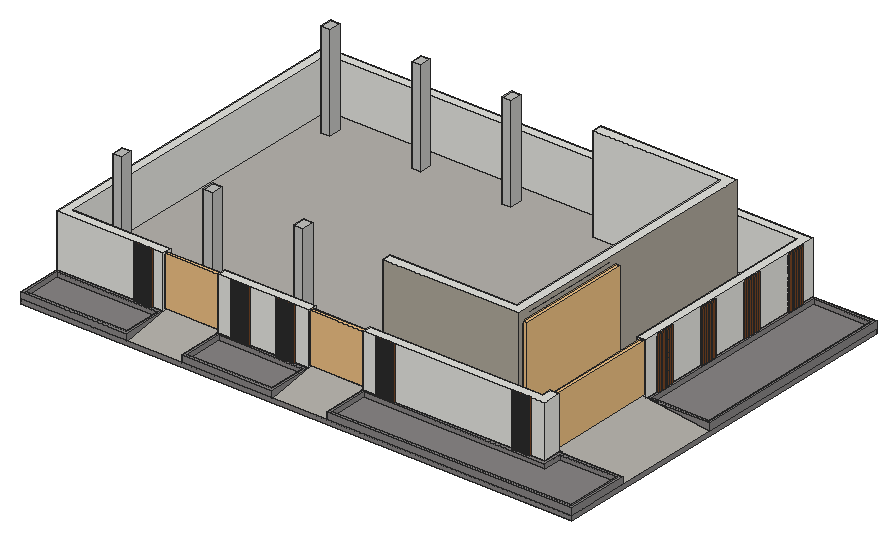
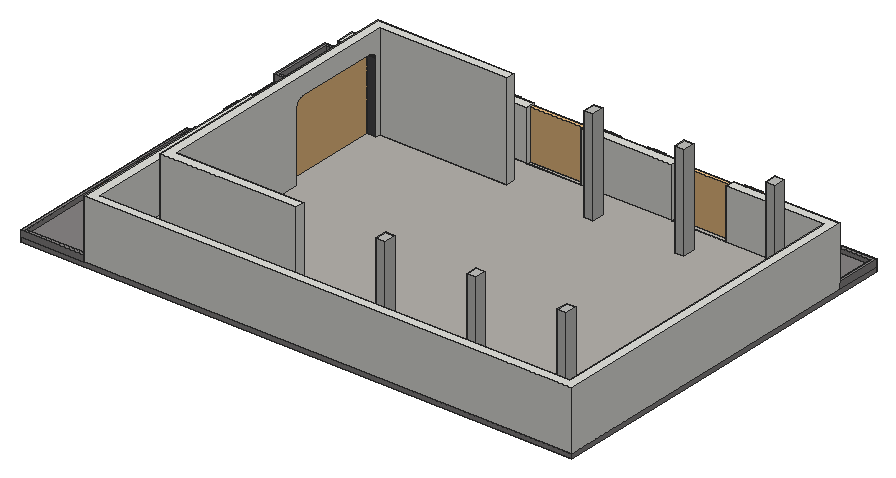
# SketchUp Ruby script. Lengths in inches.
U = 1.inch
M = Sketchup.active_model
def pt(a) = Geom::Point3d.new(a.map { |v| v * U })
def face(e, loops, mat)
  f = e.add_face(loops[0].map { |a| pt(a) })
  loops[1..].each { |l| e.add_face(l.map { |a| pt(a) }).erase! }
  f.material = f.back_material = mat if mat
  f
end
# faces: each face lists its corners as indices into pts; further lists are holes
def faces(e, pts, list, mat = nil) = list.each { |f| face(e, (f[0].is_a?(Array) ? f : [f]).map { |l| l.map { |i| pts[i] } }, mat) }
# xy, xz, yz: faces in a plane at the given z, y or x. An outline is a flat list of corners, or four numbers for a rectangle; further outlines are holes
def ring(l) = l.size == 4 ? [[l[0], l[1]], [l[2], l[1]], [l[2], l[3]], [l[0], l[3]]] : l.each_slice(2).to_a
def flat(e, list, mat, &to3) = list.each { |f| face(e, (f[0].is_a?(Array) ? f : [f]).map { |l| ring(l).map { |u, v| to3.(u, v) } }, mat) }
def xy(e, z, list, mat = nil) = flat(e, list, mat) { |x, y| [x, y, z] }
def xz(e, y, list, mat = nil) = flat(e, list, mat) { |x, z| [x, y, z] }
def yz(e, x, list, mat = nil) = flat(e, list, mat) { |y, z| [x, y, z] }
def lines(e, pts, list) = list.each { |a, b| e.add_line(pt(pts[a]), pt(pts[b])) }
# prism: a flat outline (further loops are holes) pulled along v
def prism(e, loops, v, mat = nil)
  f = face(e, loops, mat); d = Geom::Vector3d.new(v.map { |x| x * U })
  f.pushpull(f.normal.samedirection?(d) ? d.length : -d.length)
end
def box(e, o, s, mat = nil) = prism(e, [[o, [o[0] + s[0], o[1], o[2]], [o[0] + s[0], o[1] + s[1], o[2]], [o[0], o[1] + s[1], o[2]]]], [0, 0, s[2]], mat)
def at(x, y, z, deg = 0) = Geom::Transformation.translation(pt([x, y, z])) * Geom::Transformation.rotation(ORIGIN, Z_AXIS, deg.degrees)
def axes(o, x, y, z) = Geom::Transformation.new([*x, 0, *y, 0, *z, 0, *pt(o).to_a, 1])
def part(name) = M.definitions.add(name)
# library, detail: a bought-in or finely detailed component or shape, given as its bounding box
def library(name, o, s) = part(name).tap { |d| box(d.entities, o, s) }
def detail(e, o, s) = box(e.add_group.entities, o, s)
def put(e, d, t, mat = nil) = e.add_instance(d, t).tap { |i| i.material = mat if mat }
def group(e, t, mat = nil) = e.add_group.tap { |g| g.transformation = t; g.material = mat if mat }.entities
root = M.entities
M.materials.add("1432 AP 8245 TAR ROAD").color = [71, 72, 75]
M.materials.add("Generic").color = [172, 166, 153]
M.materials.add("W142X827B75_NILAYA IMAGINE 31756 ROLL B75").color = [192, 192, 189]
M.materials.add("[Brick Tumbled]").color = [135, 132, 132]
M.materials.add("[Tile Travertine 2 inch]").color = [181, 178, 172]
M.materials.add("[Wood Veneer 01]").color = [120, 70, 37]
c1 = part("Group128\#1")
box(c1.entities,[-12,-39,0],[2,78,1.5])
c2 = part("Group129\#1")
box(c2.entities,[-9.25,-39,0],[2,78,1.5])
c3 = part("Group130\#1")
box(c3.entities,[-6.5,-39,0],[2,78,1.5])
c4 = part("Group131\#1")
box(c4.entities,[-3.75,-39,0],[2,78,1.5])
c5 = part("Group132\#1")
box(c5.entities,[-1,-39,0],[2,78,1.5])
c6 = part("Group133\#1")
box(c6.entities,[1.75,-39,0],[2,78,1.5])
c7 = part("Group134\#1")
box(c7.entities,[4.5,-39,0],[2,78,1.5])
c8 = part("Group135\#1")
box(c8.entities,[7.25,-39,0],[2,78,1.5])
c9 = part("Group136\#1")
box(c9.entities,[10,-39,0],[2,78,1.5])
c10 = part("Group126\#1")
put(c10.entities,c1,at(0,0,0))
put(c10.entities,c2,at(0,0,0))
put(c10.entities,c3,at(0,0,0))
put(c10.entities,c4,at(0,0,0))
put(c10.entities,c5,at(0,0,0))
put(c10.entities,c6,at(0,0,0))
put(c10.entities,c7,at(0,0,0))
put(c10.entities,c8,at(0,0,0))
put(c10.entities,c9,at(0,0,0))
c11 = part("Group\#64")
put(c11.entities,c10,axes([12,0,39],[1,0,0],[0,0,1],[0,-1,0]))
c12 = part("Group\#66")
prism(c12.entities,[[[0,-72,0],[0,0,12],[0,0,0]]],[72,0,0])
c13 = library("Group\#1077",[59.37,-1.74,0],[60.38,4.74,59.75])
c14 = library("Group\#63",[0,7,0],[5,154,113])
c15 = library("Double slatted gate",[7.03,-128.55,-3.91],[5.33,99.02,60.06])
c16 = part("5")
box(c16.entities,[0,0,0],[12,16,126])
box(root,[0,0,11.79],[729,503.37,6],"[Brick Tumbled]")
g1 = group(root,at(0,0,17.79),"[Brick Tumbled]")
xy(g1,0,[[0,0,141,60],[213,0,333,60],[405,0,405,60,645,60,645,84,729,84,729,0],[645,228,729,503.37]])
xy(g1,3,[[4,4,137,56],[217,4,329,56],[409,4,725,4,725,80,649,80,649,56,409,56],[649,232,725,499.37]])
xy(g1,9,[[[0,0,141,60],[4,4,137,56]],[[213,0,333,60],[217,4,329,56]],[[405,0,729,0,729,84,645,84,645,60,405,60],[409,4,409,56,649,56,649,80,725,80,725,4]],[[645,228,729,503.37],[649,232,725,499.37]]])
xz(g1,0,[[0,0,141,9],[213,0,333,9],[405,0,729,9]])
xz(g1,4,[[4,3,137,9],[217,3,329,9],[409,3,725,9]])
xz(g1,56,[[4,3,137,9],[217,3,329,9],[409,3,649,9]])
xz(g1,60,[[0,0,141,9],[213,0,333,9],[405,0,645,9]])
xz(g1,80,[[649,3,725,9]])
xz(g1,84,[[645,0,729,9]])
xz(g1,228,[[645,0,729,9]])
xz(g1,232,[[649,3,725,9]])
xz(g1,499.37,[[649,3,725,9]])
xz(g1,503.37,[[645,0,729,9]])
yz(g1,0,[[0,0,60,9]])
yz(g1,4,[[4,3,56,9]])
yz(g1,137,[[4,3,56,9]])
yz(g1,141,[[0,0,60,9]])
yz(g1,213,[[0,0,60,9]])
yz(g1,217,[[4,3,56,9]])
yz(g1,329,[[4,3,56,9]])
yz(g1,333,[[0,0,60,9]])
yz(g1,405,[[0,0,60,9]])
yz(g1,409,[[4,3,56,9]])
yz(g1,645,[[60,0,84,9],[228,0,503.37,9]])
yz(g1,649,[[56,3,80,9],[232,3,499.37,9]])
yz(g1,725,[[4,3,80,9],[232,3,499.37,9]])
yz(g1,729,[[0,0,84,9],[228,0,503.37,9]])
g2 = group(root,at(36,96,29.79))
xy(g2,-12,[[-36,-36,-36,407.37,609,407.37,609,132,597,132,597,-12,609,-12,609,-36,369,-36,369,-24,297,-24,297,-36,177,-36,177,-24,105,-24,105,-36]])
xy(g2,0,[[-24,-24,597,395.37]],"[Tile Travertine 2 inch]")
xy(g2,66,[[-36,-36,105,-36,105,-24,-24,-24,-24,395.37,597,395.37,597,132,609,132,609,407.37,-36,407.37],[177,-36,297,-24],[369,-36,609,-36,609,-12,597,-12,597,-24,369,-24]])
xz(g2,-36,[[-36,-12,105,66],[177,-12,297,66],[369,-12,609,66]])
xz(g2,-24,[[105,-12,177,0],[297,-12,369,0],[-24,0,105,66],[177,0,297,66],[369,0,597,66]])
xz(g2,-12,[[597,-12,609,66]])
xz(g2,132,[[597,-12,609,66]])
xz(g2,395.37,[[-24,0,597,66]])
xz(g2,407.37,[[-36,-12,609,66]])
yz(g2,-36,[[-36,-12,407.37,66]])
yz(g2,-24,[[-24,0,395.37,66]])
yz(g2,105,[[-36,-12,-24,66]])
yz(g2,177,[[-36,-12,-24,66]])
yz(g2,297,[[-36,-12,-24,66]])
yz(g2,369,[[-36,-12,-24,66]])
yz(g2,597,[[-12,-12,132,0],[-24,0,-12,66],[132,0,395.37,66]])
yz(g2,609,[[-36,-12,-12,66],[132,-12,407.37,66]])
put(g2,c11,axes([387,-36,-3],[1,0,0],[0,1,0],[0,0,0.88462]),"[Wood Veneer 01]")
put(g2,c11,axes([566.875,-36,-3],[1,0,0],[0,1,0],[0,0,0.88462]),"[Wood Veneer 01]")
put(g2,c11,axes([254.875,-36,-3],[1,0,0],[0,1,0],[0,0,0.88462]),"[Wood Veneer 01]")
put(g2,c11,axes([195,-36,-3],[1,0,0],[0,1,0],[0,0,0.88462]),"[Wood Veneer 01]")
put(g2,c11,axes([67,-36,-3],[1,0,0],[0,1,0],[0,0,0.88462]),"[Wood Veneer 01]")
put(g2,c11,axes([609,150,-3],[0,1,0],[-1,0,0],[0,0,0.88462]),"[Wood Veneer 01]")
put(g2,c11,axes([609,365.37,-3],[0,1,0],[-1,0,0],[0,0,0.88462]),"[Wood Veneer 01]")
put(g2,c11,axes([609,221.79,-3],[0,1,0],[-1,0,0],[0,0,0.88462]),"[Wood Veneer 01]")
put(g2,c11,axes([609,293.58,-3],[0,1,0],[-1,0,0],[0,0,0.88462]),"[Wood Veneer 01]")
g3 = group(g2,at(597,-12,-12),"[Tile Travertine 2 inch]")
prism(g3,[[[0,144,0],[0,144,12],[96,144,0]]],[0,-144,0])
put(g2,c12,at(297,-24,-12),"[Tile Travertine 2 inch]")
put(g2,c12,at(105,-24,-12),"[Tile Travertine 2 inch]")
put(root,c13,axes([475.8,64.89,29.72],[-1.19247,0,0],[0,-1,0],[0,0,1.08855]))
put(root,c13,axes([283.8,64.89,29.72],[-1.19247,0,0],[0,-1,0],[0,0,1.08855]))
g4 = group(root,at(393,107.37,29.79))
xy(g4,0,[[0,0,0,12,168,12,168,18,180,18,180,0],[168,150,168,348,0,348,0,360,180,360,180,150]])
xy(g4,101.99,[[168,26.53,180,26.6875],[168,141.3125,180,141.47]],"1432 AP 8245 TAR ROAD")
xy(g4,102,[[168,26.84,180,27],[168,27,180,141],[168,141,180,141.16]],"1432 AP 8245 TAR ROAD")
xy(g4,126,[[0,0,180,0,180,360,0,360,0,348,168,348,168,12,0,12]])
xz(g4,0,[[0,0,180,126]],"Generic")
xz(g4,12,[[0,0,168,126]])
xz(g4,18,[[168,0,180,93],[168,93,180,93.16]],"1432 AP 8245 TAR ROAD")
xz(g4,18.01,[[168,93.3125,180,93.47]],"1432 AP 8245 TAR ROAD")
xz(g4,149.99,[[168,93.3125,180,93.47]],"1432 AP 8245 TAR ROAD")
xz(g4,150,[[168,0,180,93],[168,93,180,93.16]],"1432 AP 8245 TAR ROAD")
xz(g4,348,[[0,0,168,126]])
xz(g4,360,[[0,0,180,126]])
yz(g4,0,[[0,0,12,126],[348,0,360,126]])
yz(g4,168,[[12,0,12,126,348,126,348,0,150,0,150,93.16,149.99,93.3125,149.99,93.47,149.98,93.63,149.97,93.78,149.93,94.1,149.91,94.25,149.89,94.41,149.86,94.5625,149.83,94.72,149.77,95.02,149.73,95.18,149.61,95.63,149.46,96.08,149.4,96.23,149.34,96.37,149.28,96.52,149.16,96.8,149.09,96.95,148.95,97.23,148.87,97.36,148.71,97.64,148.55,97.9,148.28,98.29,148.1875,98.42,148.09,98.54,147.99,98.66,147.89,98.79,147.79,98.9,147.6875,99.02,147.58,99.14,147.14,99.58,147.02,99.6875,146.9,99.79,146.79,99.89,146.66,99.99,146.54,100.09,146.42,100.1875,146.29,100.28,145.9,100.55,145.64,100.71,145.36,100.87,145.23,100.95,144.95,101.09,144.8,101.16,144.52,101.28,144.37,101.34,144.23,101.4,144.08,101.46,143.63,101.61,143.18,101.73,143.02,101.77,142.72,101.83,142.5625,101.86,142.41,101.89,142.25,101.91,142.1,101.93,141.78,101.97,141.63,101.98,141.47,101.99,141.3125,101.99,141.16,102,26.84,102,26.6875,101.99,26.53,101.99,26.37,101.98,26.22,101.97,25.9,101.93,25.75,101.91,25.59,101.89,25.4375,101.86,25.28,101.83,24.98,101.77,24.82,101.73,24.37,101.61,23.92,101.46,23.77,101.4,23.63,101.34,23.48,101.28,23.2,101.16,23.05,101.09,22.77,100.95,22.64,100.87,22.36,100.71,22.1,100.55,21.71,100.28,21.58,100.1875,21.46,100.09,21.34,99.99,21.21,99.89,21.1,99.79,20.98,99.6875,20.86,99.58,20.42,99.14,20.3125,99.02,20.21,98.9,20.11,98.79,20.01,98.66,19.91,98.54,19.8125,98.42,19.72,98.29,19.45,97.9,19.29,97.64,19.13,97.36,19.05,97.23,18.91,96.95,18.84,96.8,18.72,96.52,18.66,96.37,18.6,96.23,18.54,96.08,18.39,95.63,18.27,95.18,18.23,95.02,18.17,94.72,18.14,94.5625,18.11,94.41,18.09,94.25,18.07,94.1,18.03,93.78,18.02,93.63,18.01,93.47,18.01,93.3125,18,93.16,18,0]])
yz(g4,180,[[0,0,18,0,18,93.16,18.01,93.3125,18.01,93.47,18.02,93.63,18.03,93.78,18.07,94.1,18.09,94.25,18.11,94.41,18.14,94.5625,18.17,94.72,18.23,95.02,18.27,95.18,18.39,95.63,18.54,96.08,18.6,96.23,18.66,96.37,18.72,96.52,18.84,96.8,18.91,96.95,19.05,97.23,19.13,97.36,19.29,97.64,19.45,97.9,19.72,98.29,19.8125,98.42,19.91,98.54,20.01,98.66,20.11,98.79,20.21,98.9,20.3125,99.02,20.42,99.14,20.86,99.58,20.98,99.6875,21.1,99.79,21.21,99.89,21.34,99.99,21.46,100.09,21.58,100.1875,21.71,100.28,22.1,100.55,22.36,100.71,22.64,100.87,22.77,100.95,23.05,101.09,23.2,101.16,23.48,101.28,23.63,101.34,23.77,101.4,23.92,101.46,24.37,101.61,24.82,101.73,24.98,101.77,25.28,101.83,25.4375,101.86,25.59,101.89,25.75,101.91,25.9,101.93,26.22,101.97,26.37,101.98,26.53,101.99,26.6875,101.99,26.84,102,141.16,102,141.3125,101.99,141.47,101.99,141.63,101.98,141.78,101.97,142.1,101.93,142.25,101.91,142.41,101.89,142.5625,101.86,142.72,101.83,143.02,101.77,143.18,101.73,143.63,101.61,144.08,101.46,144.23,101.4,144.37,101.34,144.52,101.28,144.8,101.16,144.95,101.09,145.23,100.95,145.36,100.87,145.64,100.71,145.9,100.55,146.29,100.28,146.42,100.1875,146.54,100.09,146.66,99.99,146.79,99.89,146.9,99.79,147.02,99.6875,147.14,99.58,147.58,99.14,147.6875,99.02,147.79,98.9,147.89,98.79,147.99,98.66,148.09,98.54,148.1875,98.42,148.28,98.29,148.55,97.9,148.71,97.64,148.87,97.36,148.95,97.23,149.09,96.95,149.16,96.8,149.28,96.52,149.34,96.37,149.4,96.23,149.46,96.08,149.61,95.63,149.73,95.18,149.77,95.02,149.83,94.72,149.86,94.5625,149.89,94.41,149.91,94.25,149.93,94.1,149.97,93.78,149.98,93.63,149.99,93.47,149.99,93.3125,150,93.16,150,0,360,0,360,126,0,126]],"Generic")
p = [[168,18.01,93.3125],[180,18.01,93.3125],[180,18,93.16],[168,18,93.16],[168,150,93.16],[180,150,93.16],
  [180,149.99,93.3125],[168,149.99,93.3125],[168,18.02,93.63],[180,18.02,93.63],[180,18.01,93.47],[168,18.01,93.47],
  [168,149.99,93.47],[180,149.99,93.47],[180,149.98,93.63],[168,149.98,93.63],[168,18.03,93.78],[180,18.03,93.78],
  [180,149.97,93.78],[168,149.97,93.78],[168,18.05,93.94],[180,18.05,93.94],[180,149.95,93.94],[168,149.95,93.94],
  [168,18.07,94.1],[180,18.07,94.1],[180,149.93,94.1],[168,149.93,94.1],[168,18.09,94.25],[180,18.09,94.25],
  [180,149.91,94.25],[168,149.91,94.25],[168,18.11,94.41],[180,18.11,94.41],[180,149.89,94.41],[168,149.89,94.41],
  [168,18.14,94.5625],[180,18.14,94.5625],[180,149.86,94.5625],[168,149.86,94.5625],[168,18.17,94.72],[180,18.17,94.72],
  [180,149.83,94.72],[168,149.83,94.72],[168,18.2,94.87],[180,18.2,94.87],[180,149.8,94.87],[168,149.8,94.87],
  [168,18.23,95.02],[180,18.23,95.02],[180,149.77,95.02],[168,149.77,95.02],[168,18.27,95.18],[180,18.27,95.18],
  [180,149.73,95.18],[168,149.73,95.18],[168,18.31,95.33],[180,18.31,95.33],[180,149.69,95.33],[168,149.69,95.33],
  [168,18.35,95.48],[180,18.35,95.48],[180,149.65,95.48],[168,149.65,95.48],[168,18.39,95.63],[180,18.39,95.63],
  [180,149.61,95.63],[168,149.61,95.63],[168,18.44,95.78],[180,18.44,95.78],[180,149.56,95.78],[168,149.56,95.78],
  [168,18.49,95.93],[180,18.49,95.93],[180,149.51,95.93],[168,149.51,95.93],[168,18.54,96.08],[180,18.54,96.08],
  [180,149.46,96.08],[168,149.46,96.08],[168,18.6,96.23],[180,18.6,96.23],[180,149.4,96.23],[168,149.4,96.23],
  [168,18.66,96.37],[180,18.66,96.37],[180,149.34,96.37],[168,149.34,96.37],[168,18.72,96.52],[180,18.72,96.52],
  [180,149.28,96.52],[168,149.28,96.52],[168,18.78,96.66],[180,18.78,96.66],[180,149.22,96.66],[168,149.22,96.66],
  [168,18.84,96.8],[180,18.84,96.8],[180,149.16,96.8],[168,149.16,96.8],[168,18.91,96.95],[180,18.91,96.95],
  [180,149.09,96.95],[168,149.09,96.95],[168,18.98,97.09],[180,18.98,97.09],[180,149.02,97.09],[168,149.02,97.09],
  [168,19.05,97.23],[180,19.05,97.23],[180,148.95,97.23],[168,148.95,97.23],[168,19.13,97.36],[180,19.13,97.36],
  [180,148.87,97.36],[168,148.87,97.36],[168,19.21,97.5],[180,19.21,97.5],[180,148.79,97.5],[168,148.79,97.5],
  [168,19.29,97.64],[180,19.29,97.64],[180,148.71,97.64],[168,148.71,97.64],[168,19.37,97.77],[180,19.37,97.77],
  [180,148.63,97.77],[168,148.63,97.77],[168,19.45,97.9],[180,19.45,97.9],[180,148.55,97.9],[168,148.55,97.9],
  [168,19.54,98.03],[180,19.54,98.03],[180,148.46,98.03],[168,148.46,98.03],[168,19.63,98.16],[180,19.63,98.16],
  [180,148.37,98.16],[168,148.37,98.16],[168,19.72,98.29],[180,19.72,98.29],[180,148.28,98.29],[168,148.28,98.29],
  [168,19.8125,98.42],[180,19.8125,98.42],[180,148.1875,98.42],[168,148.1875,98.42],[168,19.91,98.54],[180,19.91,98.54],
  [180,148.09,98.54],[168,148.09,98.54],[168,20.01,98.66],[180,20.01,98.66],[180,147.99,98.66],[168,147.99,98.66],
  [168,20.11,98.79],[180,20.11,98.79],[180,147.89,98.79],[168,147.89,98.79],[168,20.21,98.9],[180,20.21,98.9],
  [180,147.79,98.9],[168,147.79,98.9],[168,20.3125,99.02],[180,20.3125,99.02],[180,147.6875,99.02],[168,147.6875,99.02],
  [168,20.42,99.14],[180,20.42,99.14],[180,147.58,99.14],[168,147.58,99.14],[168,20.53,99.25],[180,20.53,99.25],
  [180,147.47,99.25],[168,147.47,99.25],[168,20.64,99.36],[180,20.64,99.36],[180,147.36,99.36],[168,147.36,99.36],
  [168,20.75,99.47],[180,20.75,99.47],[180,147.25,99.47],[168,147.25,99.47],[168,20.86,99.58],[180,20.86,99.58],
  [180,147.14,99.58],[168,147.14,99.58],[168,20.98,99.6875],[180,20.98,99.6875],[180,147.02,99.6875],[168,147.02,99.6875],
  [168,21.1,99.79],[180,21.1,99.79],[180,146.9,99.79],[168,146.9,99.79],[168,21.21,99.89],[180,21.21,99.89],
  [180,146.79,99.89],[168,146.79,99.89],[168,21.34,99.99],[180,21.34,99.99],[180,146.66,99.99],[168,146.66,99.99],
  [168,21.46,100.09],[180,21.46,100.09],[180,146.54,100.09],[168,146.54,100.09],[168,21.58,100.1875],[180,21.58,100.1875],
  [180,146.42,100.1875],[168,146.42,100.1875],[168,21.71,100.28],[180,21.71,100.28],[180,146.29,100.28],[168,146.29,100.28],
  [168,21.84,100.37],[180,21.84,100.37],[180,146.16,100.37],[168,146.16,100.37],[168,21.97,100.46],[180,21.97,100.46],
  [180,146.03,100.46],[168,146.03,100.46],[168,22.1,100.55],[180,22.1,100.55],[168,22.23,100.63],[180,22.23,100.63],
  [168,145.9,100.55],[180,145.9,100.55],[180,145.77,100.63],[168,145.77,100.63],[168,22.36,100.71],[180,22.36,100.71],
  [180,145.64,100.71],[168,145.64,100.71],[168,22.5,100.79],[180,22.5,100.79],[180,145.5,100.79],[168,145.5,100.79],
  [168,22.64,100.87],[180,22.64,100.87],[180,145.36,100.87],[168,145.36,100.87],[168,22.77,100.95],[180,22.77,100.95],
  [168,22.91,101.02],[180,22.91,101.02],[168,145.23,100.95],[180,145.23,100.95],[180,145.09,101.02],[168,145.09,101.02],
  [168,23.05,101.09],[180,23.05,101.09],[180,144.95,101.09],[168,144.95,101.09],[168,23.2,101.16],[180,23.2,101.16],
  [180,144.8,101.16],[168,144.8,101.16],[168,23.34,101.22],[180,23.34,101.22],[168,23.48,101.28],[180,23.48,101.28],
  [168,144.66,101.22],[180,144.66,101.22],[180,144.52,101.28],[168,144.52,101.28],[168,23.63,101.34],[180,23.63,101.34],
  [168,23.77,101.4],[180,23.77,101.4],[168,144.37,101.34],[180,144.37,101.34],[180,144.23,101.4],[168,144.23,101.4],
  [168,23.92,101.46],[180,23.92,101.46],[180,144.08,101.46],[168,144.08,101.46],[168,24.07,101.51],[180,24.07,101.51],
  [168,24.22,101.56],[180,24.22,101.56],[168,143.93,101.51],[180,143.93,101.51],[180,143.78,101.56],[168,143.78,101.56],
  [168,24.37,101.61],[180,24.37,101.61],[168,24.52,101.65],[180,24.52,101.65],[168,143.63,101.61],[180,143.63,101.61],
  [180,143.48,101.65],[168,143.48,101.65],[168,24.67,101.69],[180,24.67,101.69],[168,24.82,101.73],[180,24.82,101.73],
  [168,24.98,101.77],[180,24.98,101.77],[168,143.18,101.73],[180,143.18,101.73],[180,143.02,101.77],[168,143.02,101.77],
  [168,143.33,101.69],[180,143.33,101.69],[168,25.13,101.8],[180,25.13,101.8],[168,25.28,101.83],[180,25.28,101.83],
  [168,25.4375,101.86],[180,25.4375,101.86],[168,142.72,101.83],[180,142.72,101.83],[180,142.5625,101.86],[168,142.5625,101.86],
  [168,142.87,101.8],[180,142.87,101.8],[168,25.59,101.89],[180,25.59,101.89],[168,25.75,101.91],[180,25.75,101.91],
  [168,25.9,101.93],[180,25.9,101.93],[168,26.06,101.95],[180,26.06,101.95],[168,142.1,101.93],[180,142.1,101.93],
  [180,141.94,101.95],[168,141.94,101.95],[168,142.25,101.91],[180,142.25,101.91],[168,142.41,101.89],[180,142.41,101.89],
  [168,26.22,101.97],[180,26.22,101.97],[168,26.37,101.98],[180,26.37,101.98],[168,26.53,101.99],[180,26.53,101.99],
  [168,26.84,102],[180,26.84,102],[180,26.6875,101.99],[168,26.6875,101.99],[168,141.3125,101.99],[180,141.3125,101.99],
  [180,141.16,102],[168,141.16,102],[168,141.63,101.98],[180,141.63,101.98],[180,141.47,101.99],[168,141.47,101.99],
  [168,141.78,101.97],[180,141.78,101.97],[180,18,120],[180,150,120]]
faces(g4,p,[[0,1,2,3],[4,5,6,7],[8,9,10,11],[12,13,14,15],[16,17,9,8],[15,14,18,19],[20,21,17,16],[19,18,22,23],
  [24,25,21,20],[23,22,26,27],[28,29,25,24],[27,26,30,31],[32,33,29,28],[31,30,34,35],[36,37,33,32],[35,34,38,39],
  [40,41,37,36],[39,38,42,43],[44,45,41,40],[43,42,46,47],[48,49,45,44],[47,46,50,51],[52,53,49,48],[51,50,54,55],
  [56,57,53,52],[55,54,58,59],[60,61,57,56],[59,58,62,63],[64,65,61,60],[63,62,66,67],[68,69,65,64],[67,66,70,71],
  [72,73,69,68],[71,70,74,75],[76,77,73,72],[75,74,78,79],[80,81,77,76],[79,78,82,83],[84,85,81,80],[83,82,86,87],
  [88,89,85,84],[87,86,90,91],[92,93,89,88],[91,90,94,95],[96,97,93,92],[95,94,98,99],[100,101,97,96],[99,98,102,103],
  [104,105,101,100],[103,102,106,107],[108,109,105,104],[107,106,110,111],[112,113,109,108],[111,110,114,115],[116,117,113,112],[115,114,118,119],
  [120,121,117,116],[119,118,122,123],[124,125,121,120],[123,122,126,127],[128,129,125,124],[127,126,130,131],[132,133,129,128],[131,130,134,135],
  [136,137,133,132],[135,134,138,139],[140,141,137,136],[139,138,142,143],[144,145,141,140],[143,142,146,147],[148,149,145,144],[147,146,150,151],
  [152,153,149,148],[151,150,154,155],[156,157,153,152],[155,154,158,159],[160,161,157,156],[159,158,162,163],[164,165,161,160],[163,162,166,167],
  [168,169,165,164],[167,166,170,171],[172,173,169,168],[171,170,174,175],[176,177,173,172],[175,174,178,179],[180,181,177,176],[179,178,182,183],
  [184,185,181,180],[183,182,186,187],[188,189,185,184],[187,186,190,191],[192,193,189,188],[191,190,194,195],[196,197,193,192],[195,194,198,199],
  [200,201,197,196],[199,198,202,203],[204,205,201,200],[203,202,206,207],[208,209,205,204],[207,206,210,211],[212,213,209,208],[211,210,214,215],
  [216,217,213,212],[215,214,218,219],[220,221,217,216],[219,218,222,223],[224,225,221,220],[226,227,225,224],[228,229,230,231],[223,222,229,228],
  [232,233,227,226],[231,230,234,235],[236,237,233,232],[235,234,238,239],[240,241,237,236],[239,238,242,243],[244,245,241,240],[246,247,245,244],
  [248,249,250,251],[243,242,249,248],[252,253,247,246],[251,250,254,255],[256,257,253,252],[255,254,258,259],[260,261,257,256],[262,263,261,260],
  [264,265,266,267],[259,258,265,264],[268,269,263,262],[270,271,269,268],[272,273,274,275],[267,266,273,272],[276,277,271,270],[275,274,278,279],
  [280,281,277,276],[282,283,281,280],[284,285,286,287],[279,278,285,284],[288,289,283,282],[290,291,289,288],[292,293,294,295],[287,286,293,292],
  [296,297,291,290],[298,299,297,296],[300,301,299,298],[302,303,304,305],[306,307,303,302],[295,294,307,306],[308,309,301,300],[310,311,309,308],
  [312,313,311,310],[314,315,316,317],[318,319,315,314],[305,304,319,318],[320,321,313,312],[322,323,321,320],[324,325,323,322],[326,327,325,324],
  [328,329,330,331],[332,333,329,328],[334,335,333,332],[317,316,335,334],[336,337,327,326],[338,339,337,336],[340,341,339,338],[342,343,344,345],
  [346,347,348,349],[350,351,352,353],[354,355,351,350],[331,330,355,354]],"1432 AP 8245 TAR ROAD")
lines(g4,p,[[356,357]])
put(g4,c14,at(180,0,0),"1432 AP 8245 TAR ROAD")
put(root,c15,axes([649.05,270.73,33.98],[-1,0,0],[0,1.45416,0],[0,0,1.06965]))
put(root,c16,at(36,451.37,29.79),"W142X827B75_NILAYA IMAGINE 31756 ROLL B75")
put(root,c16,at(36,107.37,29.79),"W142X827B75_NILAYA IMAGINE 31756 ROLL B75")
put(root,c16,at(156,107.37,29.79),"W142X827B75_NILAYA IMAGINE 31756 ROLL B75")
put(root,c16,at(156,451.37,29.79),"W142X827B75_NILAYA IMAGINE 31756 ROLL B75")
put(root,c16,at(276,107.37,29.79),"W142X827B75_NILAYA IMAGINE 31756 ROLL B75")
put(root,c16,at(276,451.37,29.79),"W142X827B75_NILAYA IMAGINE 31756 ROLL B75")
